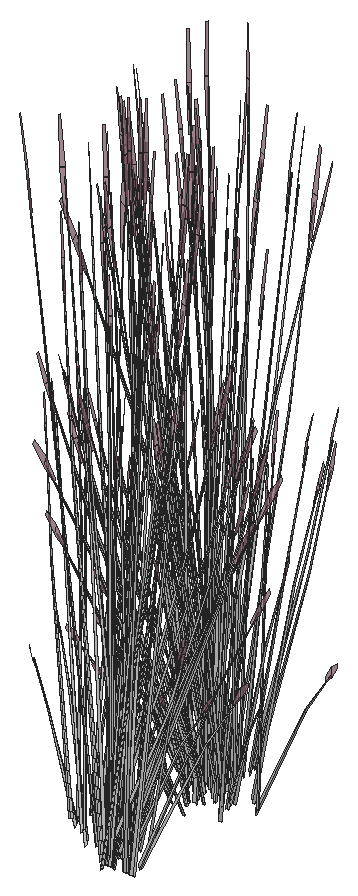
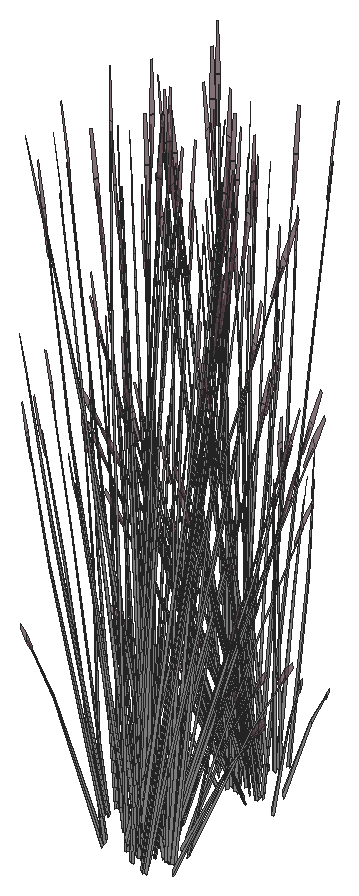
# SketchUp Ruby script. Lengths in inches.
U = 1.inch
M = Sketchup.active_model
def pt(a) = Geom::Point3d.new(a.map { |v| v * U })
def face(e, loops, mat)
  f = e.add_face(loops[0].map { |a| pt(a) })
  loops[1..].each { |l| e.add_face(l.map { |a| pt(a) }).erase! }
  f.material = f.back_material = mat if mat
  f
end
# faces: each face lists its corners as indices into pts; further lists are holes
def faces(e, pts, list, mat = nil) = list.each { |f| face(e, (f[0].is_a?(Array) ? f : [f]).map { |l| l.map { |i| pts[i] } }, mat) }
# xy, xz, yz: faces in a plane at the given z, y or x. An outline is a flat list of corners, or four numbers for a rectangle; further outlines are holes
def ring(l) = l.size == 4 ? [[l[0], l[1]], [l[2], l[1]], [l[2], l[3]], [l[0], l[3]]] : l.each_slice(2).to_a
def flat(e, list, mat, &to3) = list.each { |f| face(e, (f[0].is_a?(Array) ? f : [f]).map { |l| ring(l).map { |u, v| to3.(u, v) } }, mat) }
def xy(e, z, list, mat = nil) = flat(e, list, mat) { |x, y| [x, y, z] }
def xz(e, y, list, mat = nil) = flat(e, list, mat) { |x, z| [x, y, z] }
def yz(e, x, list, mat = nil) = flat(e, list, mat) { |y, z| [x, y, z] }
def lines(e, pts, list) = list.each { |a, b| e.add_line(pt(pts[a]), pt(pts[b])) }
# prism: a flat outline (further loops are holes) pulled along v
def prism(e, loops, v, mat = nil)
  f = face(e, loops, mat); d = Geom::Vector3d.new(v.map { |x| x * U })
  f.pushpull(f.normal.samedirection?(d) ? d.length : -d.length)
end
def box(e, o, s, mat = nil) = prism(e, [[o, [o[0] + s[0], o[1], o[2]], [o[0] + s[0], o[1] + s[1], o[2]], [o[0], o[1] + s[1], o[2]]]], [0, 0, s[2]], mat)
def at(x, y, z, deg = 0) = Geom::Transformation.translation(pt([x, y, z])) * Geom::Transformation.rotation(ORIGIN, Z_AXIS, deg.degrees)
def axes(o, x, y, z) = Geom::Transformation.new([*x, 0, *y, 0, *z, 0, *pt(o).to_a, 1])
def part(name) = M.definitions.add(name)
# library, detail: a bought-in or finely detailed component or shape, given as its bounding box
def library(name, o, s) = part(name).tap { |d| box(d.entities, o, s) }
def detail(e, o, s) = box(e.add_group.entities, o, s)
def put(e, d, t, mat = nil) = e.add_instance(d, t).tap { |i| i.material = mat if mat }
def group(e, t, mat = nil) = e.add_group.tap { |g| g.transformation = t; g.material = mat if mat }.entities
root = M.entities
M.materials.add("LightPink_Translucent").color = [144, 107, 117]
M.materials["LightPink_Translucent"].alpha = 0.75
M.materials.add("[_0053_Ivory_]").color = [200, 200, 200]
c1 = part("blade")
p = [[2.15,0.21,22],[0,0.17,0],[0.09,0.45,0],[2.18,0.31,22],[2.29,0.31,22],[0.38,0.45,0],
  [2.48,0.24,33],[2.49,0.24,33],[2.48,0.22,33]]
faces(c1.entities,p,[[0,1,2,3],[4,5,2,3],[6,3,4,7],[8,0,3,6]])
c2 = part("seeds")
p = [[0.3,-0.1,1.38],[-0.01,-0.03,1.59],[-0.01,-0.03,0.03],[0.14,-0.07,-0.07],[0.29,-0.03,3],[0.15,0.01,3.11]]
faces(c2.entities,p,[[0,1,2,3],[1,0,4,5]],"LightPink_Translucent")
c3 = part("blade with seeds")
put(c3.entities,c1,at(0,0,0))
put(c3.entities,c2,axes([2.4,0.25,30.99],[1.5799,-0.05474,1.17369],[-0.12525,1.92788,0.29478],[-0.07173,-0.02425,1.56792]))
put(root,c3,axes([644.74,139.04,128.86],[0.36485,0.52782,-0.44739],[-0.55265,0.37168,0.21531],[0.11807,0.06531,1.43643]),"[_0053_Ivory_]")
put(root,c3,axes([647.21,141.27,130.58],[-0.11624,-0.52862,-0.03492],[0.54943,-0.12153,-0.15832],[0.11473,0.03351,0.52218]),"[_0053_Ivory_]")
put(root,c3,axes([642.47,141.74,129.03],[-0.37973,0.63014,0],[-0.6353,-0.35142,-0.51607],[-0.14469,-0.08004,1.63711]),"[_0053_Ivory_]")
put(root,c3,axes([646.35,139.55,129.13],[0,-0.62885,0.49651],[0.67951,0,0],[0,0.14322,1.57504]),"[_0053_Ivory_]")
put(root,c3,axes([644.65,140.02,129.37],[0.65953,-0.03882,0.44739],[0.05964,0.64439,-0.21531],[-0.11807,0.06531,1.43643]),"[_0053_Ivory_]")
put(root,c3,axes([645.06,139.36,129.27],[0.56587,-0.18339,0.1448],[0.19817,0.52368,-0.41347],[0,0.11525,1.26744]),"[_0053_Ivory_]")
put(root,c3,axes([644.06,140.33,128.86],[-0.65953,0.03882,-0.44739],[-0.05964,-0.64439,0.21531],[-0.11807,0.06531,1.43643]),"[_0053_Ivory_]")
put(root,c3,axes([647.16,140.64,129.24],[-0.14627,-0.15466,1.43002],[0.19032,-0.51164,-0.30754],[0.29594,0.06931,0.61141]),"[_0053_Ivory_]")
put(root,c3,axes([644.55,141.2,128.86],[0.61229,0.28233,0],[-0.29468,0.58663,0],[0,0,1.74954]),"[_0053_Ivory_]")
put(root,c3,axes([644.79,141.83,128.85],[-0.37499,-0.63235,-0.05142],[0.6353,-0.35142,0.51607],[-0.15655,0.0602,1.6363]),"[_0053_Ivory_]")
put(root,c3,axes([644.66,140.3,129.27],[0.44871,0.37783,0.1448],[-0.37428,0.42627,-0.41347],[-0.10418,0.05763,1.26744]),"[_0053_Ivory_]")
put(root,c3,axes([645.82,140.95,131.63],[0.60713,0.01514,-0.71045],[-0.04078,0.63759,0.08574],[0.25721,0.06729,1.00501]),"[_0053_Ivory_]")
put(root,c3,axes([645.13,141.46,129.13],[0.56842,-0.31443,0.49651],[0.33976,0.56381,0],[-0.12946,0.07161,1.57504]),"[_0053_Ivory_]")
put(root,c3,axes([644.32,140.96,128.94],[0.26406,0.72244,-0.06012],[-0.7545,0.25315,0],[0.00922,0.02523,1.72173]),"[_0053_Ivory_]")
put(root,c3,axes([644.62,141.75,128.68],[-0.56663,-0.1556,-0.30978],[0.14267,-0.54795,0.30978],[-0.11423,0.06319,1.38974]),"[_0053_Ivory_]")
put(root,c3,axes([646.81,139.66,129.03],[0.75945,0,0],[0,0.70283,-0.51607],[0,0.16007,1.63711]),"[_0053_Ivory_]")
put(root,c3,axes([646.51,140.02,128.85],[-0.75908,-0.00503,-0.04976],[0,-0.70283,0.49943],[-0.02386,0.16,1.58352]),"[_0053_Ivory_]")
put(root,c3,axes([644.86,139.41,129.32],[0.68399,0.30005,-0.29095],[-0.32934,0.63331,-0.50002],[0.0215,0.15549,1.59708]),"[_0053_Ivory_]")
put(root,c3,axes([640.09,141.74,129.42],[0.25312,-0.28501,1.1486],[0.09988,0.45119,0.84392],[-0.18292,0.08079,0.25299]),"[_0053_Ivory_]")
put(root,c3,axes([646.18,141.21,131.18],[0.34557,0.39372,-0.35414],[-0.39459,0.37271,0.4572],[0.20048,0.05671,0.87481]),"[_0053_Ivory_]")
put(root,c3,axes([646.35,140.12,128.68],[-0.42396,0.39235,-0.30978],[-0.42396,-0.39235,0.30978],[0,0.12637,1.38974]),"[_0053_Ivory_]")
put(root,c3,axes([644.52,140.16,129.32],[0.07077,0.71755,-0.29095],[-0.73712,0.04339,-0.50002],[-0.1298,0.09558,1.59708]),"[_0053_Ivory_]")
put(root,c3,axes([644.79,139.875,128.86],[-0.29468,0.56664,-0.44739],[-0.61229,-0.27271,0.21531],[0,0.13062,1.43643]),"[_0053_Ivory_]")
put(root,c3,axes([641.04,140.51,131.18],[-0.52868,0.08987,-0.35414],[-0.1396,-0.51376,0.4572],[-0.1515,0.13799,0.87481]),"[_0053_Ivory_]")
put(root,c3,axes([644.08,140.7,128.71],[-0.40909,0.47266,-0.62353],[-0.50819,-0.4286,-0.16365],[-0.16393,0.11791,1.37633]),"[_0053_Ivory_]")
put(root,c3,axes([644.81,141.5,128.98],[0.76036,0.2044,0.30756],[-0.19023,0.7306,-0.36492],[-0.12585,0.09144,1.64885]),"[_0053_Ivory_]")
put(root,c3,axes([644.75,141.99,128.67],[-0.56842,0.31443,-0.49651],[-0.33976,-0.56381,0],[-0.12946,0.07161,1.57504]),"[_0053_Ivory_]")
put(root,c3,axes([646.64,140.13,128.67],[0,0.62885,-0.49651],[-0.67951,0,0],[0,0.14322,1.57504]),"[_0053_Ivory_]")
put(root,c3,axes([644.94,140.2,130.53],[-0.2256,-0.10835,1.71376],[0.46687,-0.45453,0.13857],[0.29098,0.20505,0.73262]),"[_0053_Ivory_]")
put(root,c3,axes([645.78,141.4375,129.42],[-0.34197,-0.18082,1.1486],[0.44156,-0.18372,0.84392],[0.1191,0.15563,0.25299]),"[_0053_Ivory_]")
put(root,c3,axes([641.96,140,130.53],[0.1517,-0.19322,1.71376],[0.38303,0.52154,0.13857],[-0.26271,0.23751,0.73262]),"[_0053_Ivory_]")
put(root,c3,axes([641.48,140.57,131.33],[0.15602,0.5742,-0.51099],[-0.59087,0.10045,-0.3958],[-0.16933,0.15423,0.97773]),"[_0053_Ivory_]")
put(root,c3,axes([645.27,141.9,129.03],[0.37973,0.63014,0],[-0.6353,0.35142,-0.51607],[-0.14469,0.08004,1.63711]),"[_0053_Ivory_]")
put(root,c3,axes([645.87,142.11,128.15],[0.04425,-0.09079,1.76342],[0.55709,-0.26738,-0.26939],[0.16889,0.13839,0.30037]),"[_0053_Ivory_]")
put(root,c3,axes([644.94,139.4,129.5],[-0.01659,-0.59209,1.41272],[0.75089,0.15348,0.59816],[-0.1776,0.32398,1.3335]),"[_0053_Ivory_]")
put(root,c3,axes([645.14,140.05,128.75],[0.2227,0.57576,-0.69212],[-0.64151,0.20736,-0.18165],[0.02462,0.19497,1.52773]),"[_0053_Ivory_]")
put(root,c3,axes([640.76,142.03,128.15],[0.08147,0.06283,1.76342],[0.13814,0.58211,-0.26939],[-0.18056,0.12413,0.30037]),"[_0053_Ivory_]")
put(root,c3,axes([645,141.6875,131.33],[0.59932,-0.14948,-0.51099],[0.10484,0.56611,-0.3958],[0.16097,0.16223,0.97773]),"[_0053_Ivory_]")
put(root,c3,axes([645.83,142.26,129.32],[-0.38947,-0.01972,1.0506],[0.25721,-0.41888,0.58006],[0.15386,0.14882,0.8241]),"[_0053_Ivory_]")
put(root,c3,axes([641.84,140.48,130.53],[0.11309,-0.21615,1.71376],[0.47441,0.44731,0.13857],[-0.21402,0.27879,0.73262]),"[_0053_Ivory_]")
put(root,c3,axes([644.56,141.24,129.24],[0.01072,-0.20846,1.43002],[0.51218,-0.23285,-0.30754],[0.15811,0.2495,0.61141]),"[_0053_Ivory_]")
put(root,c3,axes([641.97,141.7,131.18],[-0.41095,0.33109,-0.35414],[-0.38901,-0.37805,0.4572],[-0.05919,0.19208,0.87481]),"[_0053_Ivory_]")
put(root,c3,axes([642.24,142.98,129.42],[-0.01572,-0.37392,1.1486],[0.39276,0.26669,0.84392],[-0.07724,0.17822,0.25299]),"[_0053_Ivory_]")
put(root,c3,axes([642.49,151.16,130.53],[0.13883,0.2019,1.71376],[-0.64153,0.16998,0.13857],[-0.14499,-0.31697,0.73262]),"[_0053_Ivory_]")
put(root,c3,axes([643.27,142.09,128.15],[0.09829,-0.03422,1.76342],[0.59126,0.18834,-0.26939],[0.01729,0.21228,0.30037]),"[_0053_Ivory_]")
put(root,c3,axes([644.98,150.86,129.24],[-0.17264,0.12729,1.43002],[-0.51703,-0.22279,-0.30754],[0.09584,-0.27707,0.61141]),"[_0053_Ivory_]")
put(root,c3,axes([644.2,151.31,131.63],[-0.28988,-0.51132,-0.71045],[0.59671,-0.28496,0.08574],[-0.06778,-0.24706,1.00501]),"[_0053_Ivory_]")
put(root,c3,axes([642.38,141.54,131.66],[0.43478,0.42253,-0.5672],[-0.45929,0.37004,-0.43934],[-0.06615,0.21468,1.08528]),"[_0053_Ivory_]")
put(root,c3,axes([642.3125,150.62,129.24],[-0.03678,0.20572,1.43002],[-0.53767,0.17221,-0.30754],[-0.12568,-0.26589,0.61141]),"[_0053_Ivory_]")
put(root,c3,axes([641.91,142.17,129.48],[0.55175,-0.11136,0.06507],[0.12684,0.44864,-0.86304],[-0.03498,0.22711,0.7736]),"[_0053_Ivory_]")
put(root,c3,axes([643.67,141.95,131.33],[0.59704,0.15764,-0.51099],[-0.20464,0.54049,-0.3958],[0.05475,0.21761,0.97773]),"[_0053_Ivory_]")
put(root,c3,axes([644.01,140.83,130.53],[-0.13883,-0.2019,1.71376],[0.64153,-0.16998,0.13857],[0.14499,0.31697,0.73262]),"[_0053_Ivory_]")
put(root,c3,axes([643.7,150.17,128.15],[-0.10187,0.02266,1.76342],[-0.56336,-0.25503,-0.26939],[0.00945,-0.21273,0.30037]),"[_0053_Ivory_]")
put(root,c3,axes([643.4,142.28,131.18],[-0.1831,0.48359,-0.35414],[-0.53419,-0.14105,0.4572],[0.04898,0.1947,0.87481]),"[_0053_Ivory_]")
put(root,c3,axes([645.4,151.81,131.63],[0.0158,-0.58168,-0.71045],[0.66548,0.03907,0.08574],[0.07023,-0.24643,1.00501]),"[_0053_Ivory_]")
put(root,c3,axes([642.25,141.35,131.99],[-0.0158,0.58168,-0.7886],[-0.66548,-0.03907,0.09517],[-0.07023,0.24643,1.11556]),"[_0053_Ivory_]")
put(root,c3,axes([644.25,150.87,131.18],[0.1831,-0.48359,-0.35414],[0.53419,0.14105,0.4572],[-0.04898,-0.1947,0.87481]),"[_0053_Ivory_]")
put(root,c3,axes([644.65,151.51,130.53],[-0.11309,0.21615,1.71376],[-0.47441,-0.44731,0.13857],[0.21402,-0.27879,0.73262]),"[_0053_Ivory_]")
put(root,c3,axes([642.88,140.93,130.53],[-0.01487,-0.24136,1.71376],[0.64429,0.16012,0.13857],[-0.03985,0.34396,0.73262]),"[_0053_Ivory_]")
put(root,c3,axes([643.98,151.2,131.33],[-0.59704,-0.15764,-0.51099],[0.20464,-0.54049,-0.3958],[-0.05475,-0.21761,0.97773]),"[_0053_Ivory_]")
put(root,c3,axes([644.35,149.85,129.42],[0.07791,0.3667,1.1486],[-0.43222,-0.2031,0.84392],[0.04651,-0.18776,0.25299]),"[_0053_Ivory_]")
put(root,c3,axes([645.27,151.61,131.33],[-0.43478,-0.42253,-0.51099],[0.45929,-0.37004,-0.3958],[0.06615,-0.21468,0.97773]),"[_0053_Ivory_]")
put(root,c3,axes([643.46,141.85,131.63],[0.28988,0.51132,-0.71045],[-0.59671,0.28496,0.08574],[0.06778,0.24706,1.00501]),"[_0053_Ivory_]")
put(root,c3,axes([641.78,142.65,129.24],[0.19166,-0.0992,1.43002],[0.4732,0.29912,-0.30754],[-0.14084,0.25882,0.61141]),"[_0053_Ivory_]")
put(root,c3,axes([645.68,151.46,131.18],[0.41095,-0.33109,-0.35414],[0.38901,0.37805,0.4572],[0.05919,-0.19208,0.87481]),"[_0053_Ivory_]")
put(root,c3,axes([642.125,150.29,129.42],[0.31682,0.21887,1.1486],[-0.4614,0.13157,0.84392],[-0.09872,-0.16821,0.25299]),"[_0053_Ivory_]")
put(root,c3,axes([642.89,151.45,131.63],[-0.51789,-0.30395,-0.71045],[0.36805,-0.53263,0.08574],[-0.18764,-0.18149,1.00501]),"[_0053_Ivory_]")
put(root,c3,axes([642.71,151.05,131.18],[-0.0938,-0.50652,-0.35414],[0.53623,-0.13375,0.4572],[-0.14403,-0.14515,0.87481]),"[_0053_Ivory_]")
put(root,c3,axes([642.03,142.17,130.02],[0.01334,-0.32463,1.54345],[0.60018,0.17147,0.21329],[-0.052,0.34598,0.72882]),"[_0053_Ivory_]")
put(root,c3,axes([641.875,150.95,128.15],[-0.05883,0.08284,1.76342],[-0.59454,0.17861,-0.26939],[-0.14363,-0.16248,0.30037]),"[_0053_Ivory_]")
put(root,c3,axes([642.86,153.23,128.75],[-0.24943,-0.64486,-0.69835],[0.71849,-0.23224,-0.18329],[-0.02757,-0.21836,1.54149]),"[_0053_Ivory_]")
put(root,c3,axes([646.19,151.26,128.15],[-0.0909,-0.04954,1.76342],[-0.2335,-0.55347,-0.26939],[0.15752,-0.1502,0.30037]),"[_0053_Ivory_]")
put(root,c3,axes([642.65,151.47,131.33],[-0.59932,0.14948,-0.51099],[-0.10484,-0.56611,-0.3958],[-0.16097,-0.16223,0.97773]),"[_0053_Ivory_]")
put(root,c3,axes([646.1875,152.82,131.63],[0.31725,-0.49618,-0.71045],[0.55593,0.35263,0.08574],[0.18942,-0.17977,1.00501]),"[_0053_Ivory_]")
put(root,c3,axes([642.76,151.37,129.03],[-0.37973,-0.63014,0],[0.6353,-0.35142,-0.51607],[0.14469,-0.08004,1.63711]),"[_0053_Ivory_]")
put(root,c3,axes([646.17,152.59,131.33],[-0.15602,-0.5742,-0.51099],[0.59087,-0.10045,-0.3958],[0.16933,-0.15423,0.97773]),"[_0053_Ivory_]")
put(root,c3,axes([643.59,150.61,128.78],[-0.4197,0.36076,-0.03893],[-0.38456,-0.39511,-0.17649],[-0.02707,-0.11196,0.58215]),"[_0053_Ivory_]")
put(root,c3,axes([644.13,154.89,129.98],[0.52485,0.25358,1.51261],[-0.51417,0.54629,0.59816],[-0.23031,-0.32378,1.26806]),"[_0053_Ivory_]")
put(root,c3,axes([641.39,153.14,128.67],[0,-0.62885,-0.49651],[0.67951,0,0],[0,-0.14322,1.57504]),"[_0053_Ivory_]")
put(root,c3,axes([643.27,151.28,128.67],[0.56842,-0.31443,-0.49651],[0.33976,0.56381,0],[0.12946,-0.07161,1.57504]),"[_0053_Ivory_]")
put(root,c3,axes([646.65,152.36,129.24],[-0.21697,-0.01863,1.43002],[-0.22228,-0.49966,-0.30754],[0.26655,-0.14135,0.61141]),"[_0053_Ivory_]")
put(root,c3,axes([643.95,152.57,128.71],[0.40909,-0.47266,-0.62353],[0.50819,0.4286,-0.16365],[0.16393,-0.11791,1.37633]),"[_0053_Ivory_]")
put(root,c3,axes([646.9,151.44,129.42],[-0.2023,0.32011,1.1486],[-0.17388,-0.43009,0.84392],[0.16708,-0.10777,0.25299]),"[_0053_Ivory_]")
put(root,c3,axes([646.61,152.65,131.18],[0.52868,-0.08987,-0.35414],[0.1396,0.51376,0.4572],[0.1515,-0.13799,0.87481]),"[_0053_Ivory_]")
put(root,c3,axes([643.24,153.39,128.86],[0.29468,-0.56664,-0.44739],[0.61229,0.27271,0.21531],[0,-0.13062,1.43643]),"[_0053_Ivory_]")
put(root,c3,axes([641.47,151.94,131.18],[-0.34557,-0.39372,-0.35414],[0.39459,-0.37271,0.4572],[-0.20048,-0.05671,0.87481]),"[_0053_Ivory_]")
put(root,c3,axes([643.5,153.11,129.32],[-0.07077,-0.71755,-0.29095],[0.73712,-0.04339,-0.50002],[0.1298,-0.09558,1.59708]),"[_0053_Ivory_]")
put(root,c3,axes([641.68,153.15,128.68],[0.42396,-0.39235,-0.30978],[0.42396,0.39235,0.30978],[0,-0.12637,1.38974]),"[_0053_Ivory_]")
put(root,c3,axes([641.51,151.27,128.78],[-0.1752,0.51349,-0.03893],[-0.53924,-0.15795,-0.17649],[-0.08187,-0.08399,0.58215]),"[_0053_Ivory_]")
put(root,c3,axes([643.16,153.86,129.32],[-0.68399,-0.30005,-0.29095],[0.32934,-0.63331,-0.50002],[-0.0215,-0.15549,1.59708]),"[_0053_Ivory_]")
put(root,c3,axes([641.22,153.61,129.03],[-0.75945,0,0],[0,-0.70283,-0.51607],[0,-0.16007,1.63711]),"[_0053_Ivory_]")
put(root,c3,axes([643.41,151.52,128.68],[0.56663,0.1556,-0.30978],[-0.14267,0.54795,0.30978],[0.11423,-0.06319,1.38974]),"[_0053_Ivory_]")
put(root,c3,axes([641.8,153.43,128.98],[-0.56493,0.5287,0.30756],[-0.56528,-0.52313,-0.36492],[-0.01973,-0.15014,1.64885]),"[_0053_Ivory_]")
put(root,c3,axes([643.6,153.68,129.09],[0.68433,0.30479,0.24065],[-0.32934,0.63331,0.50002],[0,-0.14599,1.60543]),"[_0053_Ivory_]")
put(root,c3,axes([643.33,154.53,129.09],[0.16098,-0.74515,-0.23429],[0.76326,0.12989,0.51271],[-0.13337,-0.1029,1.5644]),"[_0053_Ivory_]")
put(root,c3,axes([640.64,152.88,129.42],[0.38775,-0.045,1.1486],[-0.24596,0.39648,0.84392],[-0.19161,-0.05948,0.25299]),"[_0053_Ivory_]")
put(root,c3,axes([643.38,153.25,129.37],[-0.65953,0.03882,0.44739],[-0.05964,-0.64439,-0.21531],[0.11807,-0.06531,1.43643]),"[_0053_Ivory_]")
put(root,c3,axes([641.68,153.72,129.13],[0,0.62885,0.49651],[-0.67951,0,0],[0,-0.14322,1.57504]),"[_0053_Ivory_]")
put(root,c3,axes([646.45,153.86,131.33],[0.16454,-0.57202,-0.51099],[0.56413,0.19607,-0.3958],[0.22713,-0.05245,0.97773]),"[_0053_Ivory_]")
put(root,c3,axes([645.55,151.53,129.03],[0.37973,-0.63014,0],[0.6353,0.35142,-0.51607],[0.14469,0.08004,1.63711]),"[_0053_Ivory_]")
put(root,c3,axes([643.28,154.23,128.86],[-0.36485,-0.52782,-0.44739],[0.55265,-0.37168,0.21531],[-0.11807,-0.06531,1.43643]),"[_0053_Ivory_]")
put(root,c3,axes([643.36,153.48,129.01],[0.26406,0.70318,0.45755],[-0.7545,0.24452,0.17955],[0.00922,-0.12921,1.58856]),"[_0053_Ivory_]")
put(root,c3,axes([647.05,154.02,128.64],[-0.39118,0.07547,1.41583],[-0.06226,-0.6007,0.08104],[0.27398,-0.09092,0.80566]),"[_0053_Ivory_]")
put(root,c3,axes([647.76,153.49,128.91],[-0.37654,-0.40212,-0.06488],[0.4124,-0.36845,-0.29416],[0.11685,-0.02594,0.97024]),"[_0053_Ivory_]")
put(root,c3,axes([643.22,154.04,129.37],[-0.29468,0.56664,0.44739],[-0.61229,-0.27271,-0.21531],[0,-0.13062,1.43643]),"[_0053_Ivory_]")
put(root,c3,axes([644.31,153.54,128.86],[0,-0.72763,0],[0.75945,0,0],[0,0,1.79456]),"[_0053_Ivory_]")
put(root,c3,axes([645.23,151.86,129.13],[-0.56842,-0.31443,0.49651],[0.33976,-0.56381,0],[0.12946,0.07161,1.57504]),"[_0053_Ivory_]")
put(root,c3,axes([646.34,154.07,131.63],[0.53369,-0.27773,-0.71045],[0.29743,0.5717,0.08574],[0.25786,-0.06494,1.00501]),"[_0053_Ivory_]")
put(root,c3,axes([642.95,154.43,128.71],[-0.63179,-0.1031,-0.62353],[0.13332,-0.63596,-0.16365],[-0.18854,-0.07706,1.37633]),"[_0053_Ivory_]")
put(root,c3,axes([643.95,153.08,129.01],[-0.50358,0.57069,0.45755],[-0.59827,-0.50377,0.17955],[0.1214,-0.05695,1.58856]),"[_0053_Ivory_]")
put(root,c3,axes([644.5,154.11,128.95],[-0.56493,-0.54126,-0.06131],[0.56528,-0.54159,0],[-0.01973,-0.0189,1.75571]),"[_0053_Ivory_]")
put(root,c3,axes([643.07,152.14,129.13],[-0.17545,0.62497,0.17642],[-0.64204,-0.17686,0.35086],[0.11091,-0.00304,1.60407]),"[_0053_Ivory_]")
put(root,c3,axes([642.81,152.65,128.25],[-0.59782,0.25177,1.28929],[-0.19028,-0.72239,0.50096],[0.36709,0.01202,1.46642]),"[_0053_Ivory_]")
put(root,c3,axes([644.41,152.84,129.27],[0.11717,-0.56122,0.1448],[0.57245,0.09742,-0.41347],[0.10418,0.05763,1.26744]),"[_0053_Ivory_]")
put(root,c3,axes([643.42,154.17,129.01],[0.76764,0.13249,0.45755],[-0.15622,0.74829,0.17955],[-0.11218,-0.07226,1.58856]),"[_0053_Ivory_]")
put(root,c3,axes([647.48,153.63,128.15],[-0.03174,-0.09547,1.76342],[0.22015,-0.55846,-0.26939],[0.22208,-0.00803,0.30037]),"[_0053_Ivory_]")
put(root,c3,axes([640.92,153.53,128.15],[0.0154,0.09911,1.76342],[-0.31051,0.51756,-0.26939],[-0.22056,-0.02609,0.30037]),"[_0053_Ivory_]")
put(root,c3,axes([644.17,152.99,129.37],[-0.36485,-0.52782,0.44739],[0.55265,-0.37168,-0.21531],[0.11807,0.06531,1.43643]),"[_0053_Ivory_]")
put(root,c3,axes([642.28,155.4,128.68],[-0.14267,-0.54795,-0.30978],[0.56663,-0.1556,0.30978],[-0.11423,-0.06319,1.38974]),"[_0053_Ivory_]")
put(root,c3,axes([643.01,155.37,129.13],[0.65264,-0.16691,0.17642],[0.16115,0.62115,0.35086],[-0.05821,-0.0905,1.60407]),"[_0053_Ivory_]")
put(root,c3,axes([644.35,153.02,129.32],[0.61322,-0.4175,-0.29095],[0.40778,0.58992,-0.50002],[0.1513,0.05991,1.59708]),"[_0053_Ivory_]")
put(root,c3,axes([646.79,154.12,131.18],[0.50475,0.17543,-0.35414],[-0.14722,0.5118,0.4572],[0.20322,-0.04693,0.87481]),"[_0053_Ivory_]")
put(root,c3,axes([642.125,155.63,128.67],[-0.56842,-0.31443,-0.49651],[0.33976,-0.56381,0],[-0.12946,-0.07161,1.57504]),"[_0053_Ivory_]")
put(root,c3,axes([645.9,151.91,128.67],[0.56842,0.31443,-0.49651],[-0.33976,0.56381,0],[0.12946,0.07161,1.57504]),"[_0053_Ivory_]")
put(root,c3,axes([644.82,153.71,128.86],[0.67951,0,0],[0,0.65103,0],[0,0,1.78407]),"[_0053_Ivory_]")
put(root,c3,axes([643.67,154.52,129.32],[-0.61322,0.4175,-0.29095],[-0.40778,-0.58992,-0.50002],[-0.1513,-0.05991,1.59708]),"[_0053_Ivory_]")
